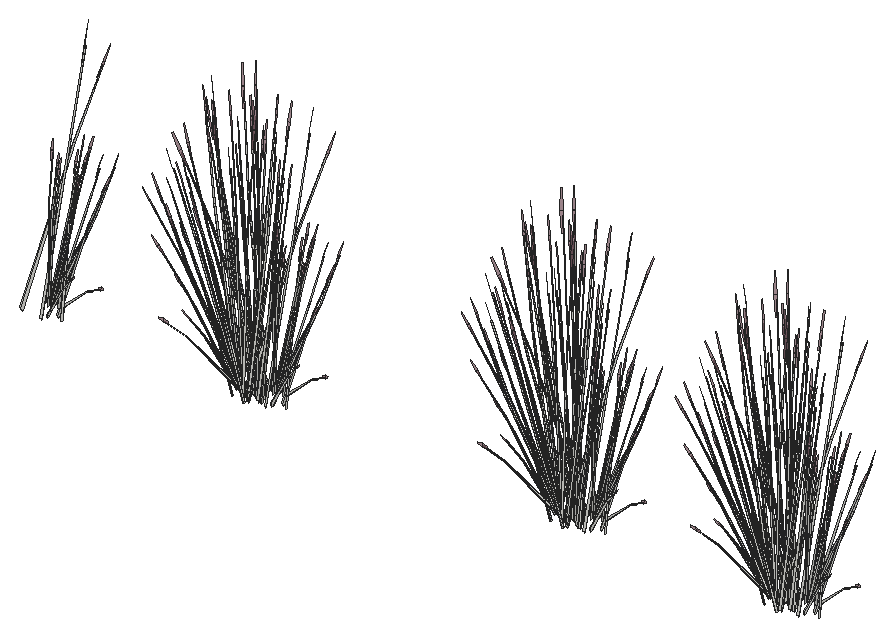
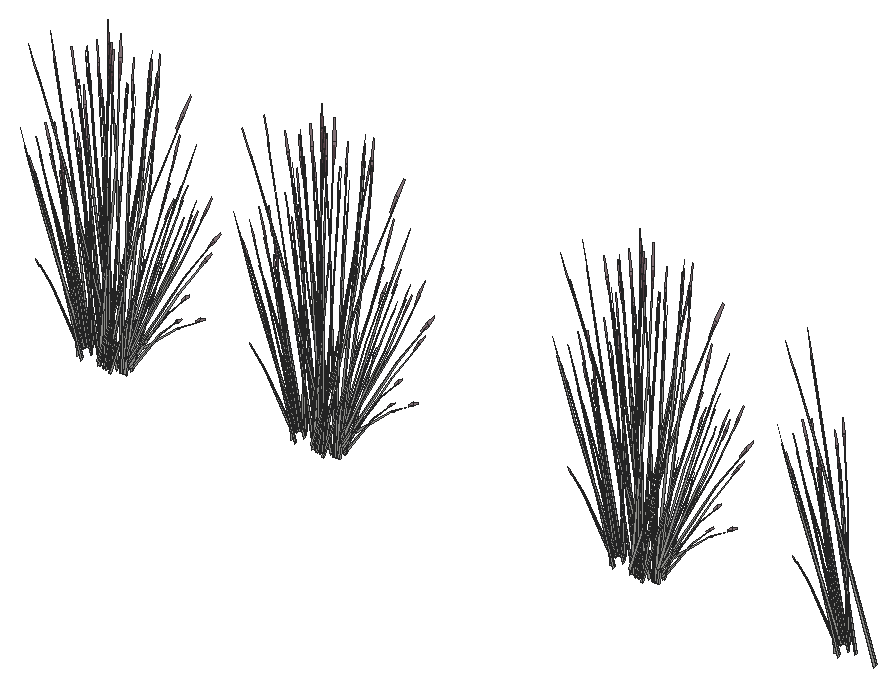
# SketchUp Ruby script. Lengths in inches.
U = 1.inch
M = Sketchup.active_model
def pt(a) = Geom::Point3d.new(a.map { |v| v * U })
def face(e, loops, mat)
  f = e.add_face(loops[0].map { |a| pt(a) })
  loops[1..].each { |l| e.add_face(l.map { |a| pt(a) }).erase! }
  f.material = f.back_material = mat if mat
  f
end
# faces: each face lists its corners as indices into pts; further lists are holes
def faces(e, pts, list, mat = nil) = list.each { |f| face(e, (f[0].is_a?(Array) ? f : [f]).map { |l| l.map { |i| pts[i] } }, mat) }
# xy, xz, yz: faces in a plane at the given z, y or x. An outline is a flat list of corners, or four numbers for a rectangle; further outlines are holes
def ring(l) = l.size == 4 ? [[l[0], l[1]], [l[2], l[1]], [l[2], l[3]], [l[0], l[3]]] : l.each_slice(2).to_a
def flat(e, list, mat, &to3) = list.each { |f| face(e, (f[0].is_a?(Array) ? f : [f]).map { |l| ring(l).map { |u, v| to3.(u, v) } }, mat) }
def xy(e, z, list, mat = nil) = flat(e, list, mat) { |x, y| [x, y, z] }
def xz(e, y, list, mat = nil) = flat(e, list, mat) { |x, z| [x, y, z] }
def yz(e, x, list, mat = nil) = flat(e, list, mat) { |y, z| [x, y, z] }
def lines(e, pts, list) = list.each { |a, b| e.add_line(pt(pts[a]), pt(pts[b])) }
# prism: a flat outline (further loops are holes) pulled along v
def prism(e, loops, v, mat = nil)
  f = face(e, loops, mat); d = Geom::Vector3d.new(v.map { |x| x * U })
  f.pushpull(f.normal.samedirection?(d) ? d.length : -d.length)
end
def box(e, o, s, mat = nil) = prism(e, [[o, [o[0] + s[0], o[1], o[2]], [o[0] + s[0], o[1] + s[1], o[2]], [o[0], o[1] + s[1], o[2]]]], [0, 0, s[2]], mat)
def at(x, y, z, deg = 0) = Geom::Transformation.translation(pt([x, y, z])) * Geom::Transformation.rotation(ORIGIN, Z_AXIS, deg.degrees)
def axes(o, x, y, z) = Geom::Transformation.new([*x, 0, *y, 0, *z, 0, *pt(o).to_a, 1])
def part(name) = M.definitions.add(name)
# library, detail: a bought-in or finely detailed component or shape, given as its bounding box
def library(name, o, s) = part(name).tap { |d| box(d.entities, o, s) }
def detail(e, o, s) = box(e.add_group.entities, o, s)
def put(e, d, t, mat = nil) = e.add_instance(d, t).tap { |i| i.material = mat if mat }
def group(e, t, mat = nil) = e.add_group.tap { |g| g.transformation = t; g.material = mat if mat }.entities
root = M.entities
M.materials.add("LightPink_Translucent").color = [144, 107, 117]
M.materials["LightPink_Translucent"].alpha = 0.75
c1 = part("blade")
p = [[2.15,0.21,22],[0,0.17,0],[0.09,0.45,0],[2.18,0.31,22],[2.29,0.31,22],[0.38,0.45,0],
  [2.48,0.24,33],[2.49,0.24,33],[2.48,0.22,33]]
faces(c1.entities,p,[[0,1,2,3],[4,5,2,3],[6,3,4,7],[8,0,3,6]])
c2 = part("seeds")
p = [[0.3,-0.1,1.38],[-0.01,-0.03,1.59],[-0.01,-0.03,0.03],[0.14,-0.07,-0.07],[0.29,-0.03,3],[0.15,0.01,3.11]]
faces(c2.entities,p,[[0,1,2,3],[1,0,4,5]],"LightPink_Translucent")
c3 = part("blade with seeds")
put(c3.entities,c1,at(0,0,0))
put(c3.entities,c2,axes([2.4,0.25,30.99],[1.5799,-0.05474,1.17369],[-0.12525,1.92788,0.29478],[-0.07173,-0.02425,1.56792]))
put(root,c3,axes([842.6875,480.84,4.49],[0.24005,-0.25798,-0.35523],[0.42065,0.18334,0.04287],[0.14333,-0.09347,0.5025]))
put(root,c3,axes([783.8125,480.08,3.1875],[-0.28732,-0.32763,0],[0.4807,-0.18271,-0.25804],[0.10948,-0.04161,0.81856]))
put(root,c3,axes([817.51,480.08,3.1875],[-0.28732,-0.32763,0],[0.4807,-0.18271,-0.25804],[0.10948,-0.04161,0.81856]))
put(root,c3,axes([840.09,480.08,3.1875],[-0.28732,-0.32763,0],[0.4807,-0.18271,-0.25804],[0.10948,-0.04161,0.81856]))
put(root,c3,axes([762.63,480.72,4.34],[-0.11806,-0.29854,-0.25549],[0.44709,-0.05222,-0.1979],[0.12812,-0.08019,0.48886]))
put(root,c3,axes([786.4,480.72,4.34],[-0.11806,-0.29854,-0.25549],[0.44709,-0.05222,-0.1979],[0.12812,-0.08019,0.48886]))
put(root,c3,axes([820.09,480.72,4.34],[-0.11806,-0.29854,-0.25549],[0.44709,-0.05222,-0.1979],[0.12812,-0.08019,0.48886]))
put(root,c3,axes([842.68,480.72,4.34],[-0.11806,-0.29854,-0.25549],[0.44709,-0.05222,-0.1979],[0.12812,-0.08019,0.48886]))
put(root,c3,axes([784.44,479.69,3.0625],[-0.31757,0.18757,-0.01946],[-0.29098,-0.20543,-0.08825],[-0.02049,-0.05821,0.29107]))
put(root,c3,axes([818.14,479.69,3.0625],[-0.31757,0.18757,-0.01946],[-0.29098,-0.20543,-0.08825],[-0.02049,-0.05821,0.29107]))
put(root,c3,axes([840.72,479.69,3.0625],[-0.31757,0.18757,-0.01946],[-0.29098,-0.20543,-0.08825],[-0.02049,-0.05821,0.29107]))
put(root,c3,axes([782.87,479.78,4.36],[-0.09888,-0.00231,0.87472],[-0.3148,0.23079,-0.13834],[-0.16797,-0.04716,0.07015]))
put(root,c3,axes([816.57,479.78,4.36],[-0.09888,-0.00231,0.87472],[-0.3148,0.23079,-0.13834],[-0.16797,-0.04716,0.07015]))
put(root,c3,axes([839.15,479.78,4.36],[-0.09888,-0.00231,0.87472],[-0.3148,0.23079,-0.13834],[-0.16797,-0.04716,0.07015]))
put(root,c3,axes([762.84,480.93,4.52],[-0.4251,-0.18028,-0.0608],[0.24491,-0.26108,-0.33747],[0.1201,-0.09075,0.51278]))
put(root,c3,axes([786.61,480.93,4.52],[-0.4251,-0.18028,-0.0608],[0.24491,-0.26108,-0.33747],[0.1201,-0.09075,0.51278]))
put(root,c3,axes([820.3,480.93,4.52],[-0.4251,-0.18028,-0.0608],[0.24491,-0.26108,-0.33747],[0.1201,-0.09075,0.51278]))
put(root,c3,axes([842.89,480.93,4.52],[-0.4251,-0.18028,-0.0608],[0.24491,-0.26108,-0.33747],[0.1201,-0.09075,0.51278]))
put(root,c3,axes([784.85,481.91,3.66],[0.39713,0.13184,0.7563],[-0.38905,0.28403,0.29908],[-0.17427,-0.16834,0.63403]))
put(root,c3,axes([818.55,481.91,3.66],[0.39713,0.13184,0.7563],[-0.38905,0.28403,0.29908],[-0.17427,-0.16834,0.63403]))
put(root,c3,axes([841.13,481.91,3.66],[0.39713,0.13184,0.7563],[-0.38905,0.28403,0.29908],[-0.17427,-0.16834,0.63403]))
put(root,c3,axes([784.02,480.13,4.53],[0.07098,0.26335,0.17707],[-0.40574,0.06954,-0.2286],[-0.10898,-0.07547,0.4374]))
put(root,c3,axes([817.71,480.13,4.53],[0.07098,0.26335,0.17707],[-0.40574,0.06954,-0.2286],[-0.10898,-0.07547,0.4374]))
put(root,c3,axes([840.3,480.13,4.53],[0.07098,0.26335,0.17707],[-0.40574,0.06954,-0.2286],[-0.10898,-0.07547,0.4374]))
put(root,c3,axes([782.77,481,3.01],[0,-0.32696,-0.24825],[0.51416,0,0],[0,-0.07447,0.78752]))
put(root,c3,axes([816.47,481,3.01],[0,-0.32696,-0.24825],[0.51416,0,0],[0,-0.07447,0.78752]))
put(root,c3,axes([839.06,481,3.01],[0,-0.32696,-0.24825],[0.51416,0,0],[0,-0.07447,0.78752]))
put(root,c3,axes([784.2,480.03,3.01],[0.4301,-0.16348,-0.24825],[0.25708,0.29314,0],[0.09796,-0.03723,0.78752]))
put(root,c3,axes([817.9,480.03,3.01],[0.4301,-0.16348,-0.24825],[0.25708,0.29314,0],[0.09796,-0.03723,0.78752]))
put(root,c3,axes([840.48,480.03,3.01],[0.4301,-0.16348,-0.24825],[0.25708,0.29314,0],[0.09796,-0.03723,0.78752]))
put(root,c3,axes([762.99,480.6,3.3],[-0.16417,-0.00968,0.71501],[-0.16819,-0.25979,-0.15377],[0.20169,-0.07349,0.3057]))
put(root,c3,axes([786.75,480.6,3.3],[-0.16417,-0.00968,0.71501],[-0.16819,-0.25979,-0.15377],[0.20169,-0.07349,0.3057]))
put(root,c3,axes([820.45,480.6,3.3],[-0.16417,-0.00968,0.71501],[-0.16819,-0.25979,-0.15377],[0.20169,-0.07349,0.3057]))
put(root,c3,axes([843.04,480.6,3.3],[-0.16417,-0.00968,0.71501],[-0.16819,-0.25979,-0.15377],[0.20169,-0.07349,0.3057]))
put(root,c3,axes([782.8,480.3,4.55],[0.37952,-0.24129,0.26881],[0.32731,0.25625,0.22165],[-0.17806,-0.04451,0.55625]))
put(root,c3,axes([816.49,480.3,4.55],[0.37952,-0.24129,0.26881],[0.32731,0.25625,0.22165],[-0.17806,-0.04451,0.55625]))
put(root,c3,axes([839.08,480.3,4.55],[0.37952,-0.24129,0.26881],[0.32731,0.25625,0.22165],[-0.17806,-0.04451,0.55625]))
put(root,c3,axes([763.89,480.85,4.35],[-0.06002,-0.00248,0.88692],[-0.24926,-0.26607,-0.08381],[0.1001,-0.08748,0.15695]))
put(root,c3,axes([787.65,480.85,4.35],[-0.06002,-0.00248,0.88692],[-0.24926,-0.26607,-0.08381],[0.1001,-0.08748,0.15695]))
put(root,c3,axes([821.35,480.85,4.35],[-0.06002,-0.00248,0.88692],[-0.24926,-0.26607,-0.08381],[0.1001,-0.08748,0.15695]))
put(root,c3,axes([843.93,480.85,4.35],[-0.06002,-0.00248,0.88692],[-0.24926,-0.26607,-0.08381],[0.1001,-0.08748,0.15695]))
put(root,c3,axes([784.71,480.7,3.03],[0.30954,-0.24575,-0.31177],[0.38452,0.22284,-0.08182],[0.12404,-0.0613,0.68817]))
put(root,c3,axes([818.41,480.7,3.03],[0.30954,-0.24575,-0.31177],[0.38452,0.22284,-0.08182],[0.12404,-0.0613,0.68817]))
put(root,c3,axes([840.99,480.7,3.03],[0.30954,-0.24575,-0.31177],[0.38452,0.22284,-0.08182],[0.12404,-0.0613,0.68817]))
put(root,c3,axes([763.18,480.12,3.38],[-0.15307,0.16644,0.5743],[-0.13157,-0.22361,0.42196],[0.12643,-0.05603,0.12649]))
put(root,c3,axes([786.94,480.12,3.38],[-0.15307,0.16644,0.5743],[-0.13157,-0.22361,0.42196],[0.12643,-0.05603,0.12649]))
put(root,c3,axes([820.64,480.12,3.38],[-0.15307,0.16644,0.5743],[-0.13157,-0.22361,0.42196],[0.12643,-0.05603,0.12649]))
put(root,c3,axes([843.23,480.12,3.38],[-0.15307,0.16644,0.5743],[-0.13157,-0.22361,0.42196],[0.12643,-0.05603,0.12649]))
put(root,c3,axes([762.96,480.75,4.26],[0.40003,-0.04673,-0.17707],[0.10563,0.26712,0.2286],[0.11464,-0.07175,0.4374]))
put(root,c3,axes([786.73,480.75,4.26],[0.40003,-0.04673,-0.17707],[0.10563,0.26712,0.2286],[0.11464,-0.07175,0.4374]))
put(root,c3,axes([820.42,480.75,4.26],[0.40003,-0.04673,-0.17707],[0.10563,0.26712,0.2286],[0.11464,-0.07175,0.4374]))
put(root,c3,axes([843.01,480.75,4.26],[0.40003,-0.04673,-0.17707],[0.10563,0.26712,0.2286],[0.11464,-0.07175,0.4374]))
put(root,c3,axes([782.97,480.3,4.37],[0.02314,-0.24862,0.03215],[0.34943,0.00682,0.2531],[-0.13385,-0.02602,0.38595]))
put(root,c3,axes([816.67,480.3,4.37],[0.02314,-0.24862,0.03215],[0.34943,0.00682,0.2531],[-0.13385,-0.02602,0.38595]))
put(root,c3,axes([839.25,480.3,4.37],[0.02314,-0.24862,0.03215],[0.34943,0.00682,0.2531],[-0.13385,-0.02602,0.38595]))
put(root,c3,axes([784.17,481.14,3.11],[0.22297,-0.29461,-0.2237],[0.4633,0.14179,0.10766],[0,-0.06791,0.71822]))
put(root,c3,axes([817.87,481.14,3.11],[0.22297,-0.29461,-0.2237],[0.4633,0.14179,0.10766],[0,-0.06791,0.71822]))
put(root,c3,axes([840.45,481.14,3.11],[0.22297,-0.29461,-0.2237],[0.4633,0.14179,0.10766],[0,-0.06791,0.71822]))
put(root,c3,axes([782.84,480.38,4.26],[-0.26148,-0.20471,-0.17707],[0.29857,-0.19378,0.2286],[-0.1517,-0.02948,0.4374]))
put(root,c3,axes([816.53,480.38,4.26],[-0.26148,-0.20471,-0.17707],[0.29857,-0.19378,0.2286],[-0.1517,-0.02948,0.4374]))
put(root,c3,axes([839.12,480.38,4.26],[-0.26148,-0.20471,-0.17707],[0.29857,-0.19378,0.2286],[-0.1517,-0.02948,0.4374]))
put(root,c3,axes([784.375,480.99,3.33],[-0.05355,-0.37308,-0.14548],[0.55775,-0.02256,-0.25001],[0.09822,-0.04969,0.79854]))
put(root,c3,axes([818.07,480.99,3.33],[-0.05355,-0.37308,-0.14548],[0.55775,-0.02256,-0.25001],[0.09822,-0.04969,0.79854]))
put(root,c3,axes([840.66,480.99,3.33],[-0.05355,-0.37308,-0.14548],[0.55775,-0.02256,-0.25001],[0.09822,-0.04969,0.79854]))
put(root,c3,axes([782.99,481.01,3.01],[0.32079,-0.20399,-0.15489],[0.32079,0.20399,0.15489],[0,-0.06571,0.69487]))
put(root,c3,axes([816.6875,481.01,3.01],[0.32079,-0.20399,-0.15489],[0.32079,0.20399,0.15489],[0,-0.06571,0.69487]))
put(root,c3,axes([839.28,481.01,3.01],[0.32079,-0.20399,-0.15489],[0.32079,0.20399,0.15489],[0,-0.06571,0.69487]))
put(root,c3,axes([782.86,480.03,3.0625],[-0.13257,0.26698,-0.01946],[-0.40802,-0.08212,-0.08825],[-0.06195,-0.04367,0.29107]))
put(root,c3,axes([816.56,480.03,3.0625],[-0.13257,0.26698,-0.01946],[-0.40802,-0.08212,-0.08825],[-0.06195,-0.04367,0.29107]))
put(root,c3,axes([839.15,480.03,3.0625],[-0.13257,0.26698,-0.01946],[-0.40802,-0.08212,-0.08825],[-0.06195,-0.04367,0.29107]))
put(root,c3,axes([762.64,480.9,4.53],[-0.40003,0.04673,0.17707],[-0.10563,-0.26712,-0.2286],[0.11464,-0.07175,0.4374]))
put(root,c3,axes([786.4,480.9,4.53],[-0.40003,0.04673,0.17707],[-0.10563,-0.26712,-0.2286],[0.11464,-0.07175,0.4374]))
put(root,c3,axes([820.09,480.9,4.53],[-0.40003,0.04673,0.17707],[-0.10563,-0.26712,-0.2286],[0.11464,-0.07175,0.4374]))
put(root,c3,axes([842.68,480.9,4.53],[-0.40003,0.04673,0.17707],[-0.10563,-0.26712,-0.2286],[0.11464,-0.07175,0.4374]))
put(root,c3,axes([784.12,481.38,3.33],[-0.51755,-0.15601,-0.14548],[0.2492,-0.32927,-0.25001],[-0.01626,-0.08084,0.79854]))
put(root,c3,axes([817.8125,481.38,3.33],[-0.51755,-0.15601,-0.14548],[0.2492,-0.32927,-0.25001],[-0.01626,-0.08084,0.79854]))
put(root,c3,axes([840.4,481.38,3.33],[-0.51755,-0.15601,-0.14548],[0.2492,-0.32927,-0.25001],[-0.01626,-0.08084,0.79854]))
put(root,c3,axes([782.65,481.25,3.1875],[-0.57465,0,0],[0,-0.36542,-0.25804],[0,-0.08323,0.81856]))
put(root,c3,axes([816.34,481.25,3.1875],[-0.57465,0,0],[0,-0.36542,-0.25804],[0,-0.08323,0.81856]))
put(root,c3,axes([838.93,481.25,3.1875],[-0.57465,0,0],[0,-0.36542,-0.25804],[0,-0.08323,0.81856]))
put(root,c3,axes([782.74,480.6,3.3],[0.08973,0.09103,0.71501],[-0.20675,0.24743,-0.15377],[-0.2123,-0.05914,0.3057]))
put(root,c3,axes([816.4375,480.6,3.3],[0.08973,0.09103,0.71501],[-0.20675,0.24743,-0.15377],[-0.2123,-0.05914,0.3057]))
put(root,c3,axes([839.02,480.6,3.3],[0.08973,0.09103,0.71501],[-0.20675,0.24743,-0.15377],[-0.2123,-0.05914,0.3057]))
put(root,c3,axes([784.3,480.16,3.01],[0.42874,0.0809,-0.15489],[-0.10795,0.28489,0.15489],[0.08643,-0.03285,0.69487]))
put(root,c3,axes([818,480.16,3.01],[0.42874,0.0809,-0.15489],[-0.10795,0.28489,0.15489],[0.08643,-0.03285,0.69487]))
put(root,c3,axes([840.58,480.16,3.01],[0.42874,0.0809,-0.15489],[-0.10795,0.28489,0.15489],[0.08643,-0.03285,0.69487]))
put(root,c3,axes([783.11,480.52,4.49],[-0.45939,-0.00787,-0.35523],[0.03085,-0.3315,0.04287],[-0.19462,-0.03498,0.5025]))
put(root,c3,axes([816.81,480.52,4.49],[-0.45939,-0.00787,-0.35523],[0.03085,-0.3315,0.04287],[-0.19462,-0.03498,0.5025]))
put(root,c3,axes([839.4,480.52,4.49],[-0.45939,-0.00787,-0.35523],[0.03085,-0.3315,0.04287],[-0.19462,-0.03498,0.5025]))
put(root,c3,axes([763,480.86,4.37],[0.31549,0.13751,0.03215],[-0.18368,0.19581,0.2531],[0.10115,-0.06331,0.38595]))
put(root,c3,axes([786.76,480.86,4.37],[0.31549,0.13751,0.03215],[-0.18368,0.19581,0.2531],[0.10115,-0.06331,0.38595]))
put(root,c3,axes([820.46,480.86,4.37],[0.31549,0.13751,0.03215],[-0.18368,0.19581,0.2531],[0.10115,-0.06331,0.38595]))
put(root,c3,axes([843.04,480.86,4.37],[0.31549,0.13751,0.03215],[-0.18368,0.19581,0.2531],[0.10115,-0.06331,0.38595]))
put(root,c3,axes([762.91,480.8,4.37],[0.11397,0.30091,0.24001],[-0.44709,0.05222,0.1979],[0.13177,-0.07077,0.49665]))
put(root,c3,axes([786.67,480.8,4.37],[0.11397,0.30091,0.24001],[-0.44709,0.05222,0.1979],[0.13177,-0.07077,0.49665]))
put(root,c3,axes([820.37,480.8,4.37],[0.11397,0.30091,0.24001],[-0.44709,0.05222,0.1979],[0.13177,-0.07077,0.49665]))
put(root,c3,axes([842.95,480.8,4.37],[0.11397,0.30091,0.24001],[-0.44709,0.05222,0.1979],[0.13177,-0.07077,0.49665]))
put(root,c3,axes([764.12,481.17,4.36],[0.06377,-0.0498,0.87472],[-0.08162,-0.30549,-0.13834],[0.16001,-0.05792,0.07015]))
put(root,c3,axes([787.88,481.17,4.36],[0.06377,-0.0498,0.87472],[-0.08162,-0.30549,-0.13834],[0.16001,-0.05792,0.07015]))
put(root,c3,axes([821.57,481.17,4.36],[0.06377,-0.0498,0.87472],[-0.08162,-0.30549,-0.13834],[0.16001,-0.05792,0.07015]))
put(root,c3,axes([844.16,481.17,4.36],[0.06377,-0.0498,0.87472],[-0.08162,-0.30549,-0.13834],[0.16001,-0.05792,0.07015]))
put(root,c3,axes([783.09,481.15,3.17],[-0.42746,0.27488,0.15378],[-0.42772,-0.27199,-0.18246],[-0.01493,-0.07806,0.82443]))
put(root,c3,axes([816.79,481.15,3.17],[-0.42746,0.27488,0.15378],[-0.42772,-0.27199,-0.18246],[-0.01493,-0.07806,0.82443]))
put(root,c3,axes([839.37,481.15,3.17],[-0.42746,0.27488,0.15378],[-0.42772,-0.27199,-0.18246],[-0.01493,-0.07806,0.82443]))
put(root,c3,axes([782.49,479.98,4.35],[0.03407,0.03263,0.88692],[-0.16424,0.29331,-0.08381],[-0.16634,0.00212,0.15695]))
put(root,c3,axes([816.19,479.98,4.35],[0.03407,0.03263,0.88692],[-0.16424,0.29331,-0.08381],[-0.16634,0.00212,0.15695]))
put(root,c3,axes([838.77,479.98,4.35],[0.03407,0.03263,0.88692],[-0.16424,0.29331,-0.08381],[-0.16634,0.00212,0.15695]))
put(root,c3,axes([784.45,481.28,3.22],[0.5178,0.15847,0.12032],[-0.2492,0.32927,0.25001],[0,-0.0759,0.80271]))
put(root,c3,axes([818.14,481.28,3.22],[0.5178,0.15847,0.12032],[-0.2492,0.32927,0.25001],[0,-0.0759,0.80271]))
put(root,c3,axes([840.73,481.28,3.22],[0.5178,0.15847,0.12032],[-0.2492,0.32927,0.25001],[0,-0.0759,0.80271]))
put(root,c3,axes([784.25,481.73,3.22],[0.1218,-0.38743,-0.11714],[0.57753,0.06753,0.25635],[-0.10091,-0.0535,0.7822]))
put(root,c3,axes([817.94,481.73,3.22],[0.1218,-0.38743,-0.11714],[0.57753,0.06753,0.25635],[-0.10091,-0.0535,0.7822]))
put(root,c3,axes([840.53,481.73,3.22],[0.1218,-0.38743,-0.11714],[0.57753,0.06753,0.25635],[-0.10091,-0.0535,0.7822]))
put(root,c3,axes([782.96,480.58,4.34],[-0.3337,0.21658,-0.25549],[-0.29224,-0.22879,-0.1979],[-0.16955,-0.03295,0.48886]))
put(root,c3,axes([816.66,480.58,4.34],[-0.3337,0.21658,-0.25549],[-0.29224,-0.22879,-0.1979],[-0.16955,-0.03295,0.48886]))
put(root,c3,axes([839.24,480.58,4.34],[-0.3337,0.21658,-0.25549],[-0.29224,-0.22879,-0.1979],[-0.16955,-0.03295,0.48886]))
put(root,c3,axes([783.21,480.49,4.53],[0.26148,0.20471,0.17707],[-0.29857,0.19378,-0.2286],[-0.1517,-0.02948,0.4374]))
put(root,c3,axes([816.9,480.49,4.53],[0.26148,0.20471,0.17707],[-0.29857,0.19378,-0.2286],[-0.1517,-0.02948,0.4374]))
put(root,c3,axes([839.49,480.49,4.53],[0.26148,0.20471,0.17707],[-0.29857,0.19378,-0.2286],[-0.1517,-0.02948,0.4374]))
put(root,c3,axes([782.21,480.87,3.38],[0.2934,-0.0234,0.5743],[-0.18611,0.20614,0.42196],[-0.14499,-0.03092,0.12649]))
put(root,c3,axes([815.9,480.87,3.38],[0.2934,-0.0234,0.5743],[-0.18611,0.20614,0.42196],[-0.14499,-0.03092,0.12649]))
put(root,c3,axes([838.49,480.87,3.38],[0.2934,-0.0234,0.5743],[-0.18611,0.20614,0.42196],[-0.14499,-0.03092,0.12649]))
put(root,c3,axes([784.28,481.0625,3.36],[-0.49904,0.02018,0.2237],[-0.04513,-0.33504,-0.10766],[0.08934,-0.03396,0.71822]))
put(root,c3,axes([817.98,481.0625,3.36],[-0.49904,0.02018,0.2237],[-0.04513,-0.33504,-0.10766],[0.08934,-0.03396,0.71822]))
put(root,c3,axes([840.5625,481.0625,3.36],[-0.49904,0.02018,0.2237],[-0.04513,-0.33504,-0.10766],[0.08934,-0.03396,0.71822]))
put(root,c3,axes([783.14,480.36,4.52],[-0.02461,0.33251,-0.0608],[-0.4659,-0.00909,-0.33747],[-0.17944,-0.0231,0.51278]))
put(root,c3,axes([816.83,480.36,4.52],[-0.02461,0.33251,-0.0608],[-0.4659,-0.00909,-0.33747],[-0.17944,-0.0231,0.51278]))
put(root,c3,axes([839.42,480.36,4.52],[-0.02461,0.33251,-0.0608],[-0.4659,-0.00909,-0.33747],[-0.17944,-0.0231,0.51278]))
put(root,c3,axes([782.99,481.31,3.24],[0,0.32696,0.24825],[-0.51416,0,0],[0,-0.07447,0.78752]))
put(root,c3,axes([816.6875,481.31,3.24],[0,0.32696,0.24825],[-0.51416,0,0],[0,-0.07447,0.78752]))
put(root,c3,axes([839.28,481.31,3.24],[0,0.32696,0.24825],[-0.51416,0,0],[0,-0.07447,0.78752]))
put(root,c3,axes([762.86,481.63,4.52],[-0.23123,-0.29606,-0.0608],[0.41039,-0.14549,-0.33747],[0.17294,-0.03906,0.51278]))
put(root,c3,axes([786.625,481.63,4.52],[-0.23123,-0.29606,-0.0608],[0.41039,-0.14549,-0.33747],[0.17294,-0.03906,0.51278]))
put(root,c3,axes([820.32,481.63,4.52],[-0.23123,-0.29606,-0.0608],[0.41039,-0.14549,-0.33747],[0.17294,-0.03906,0.51278]))
put(root,c3,axes([842.9,481.63,4.52],[-0.23123,-0.29606,-0.0608],[0.41039,-0.14549,-0.33747],[0.17294,-0.03906,0.51278]))
put(root,c3,axes([762.84,481.38,4.34],[0.1245,-0.29741,-0.25549],[0.42685,0.10194,-0.1979],[0.17186,-0.02727,0.48886]))
put(root,c3,axes([786.6,481.38,4.34],[0.1245,-0.29741,-0.25549],[0.42685,0.10194,-0.1979],[0.17186,-0.02727,0.48886]))
put(root,c3,axes([820.3,481.38,4.34],[0.1245,-0.29741,-0.25549],[0.42685,0.10194,-0.1979],[0.17186,-0.02727,0.48886]))
put(root,c3,axes([842.88,481.38,4.34],[0.1245,-0.29741,-0.25549],[0.42685,0.10194,-0.1979],[0.17186,-0.02727,0.48886]))
put(root,c3,axes([762.17,480.17,3.1875],[0.28732,-0.32763,0],[0.4807,0.18271,-0.25804],[0.10948,0.04161,0.81856]))
put(root,c3,axes([785.93,480.17,3.1875],[0.28732,-0.32763,0],[0.4807,0.18271,-0.25804],[0.10948,0.04161,0.81856]))
put(root,c3,axes([819.625,480.17,3.1875],[0.28732,-0.32763,0],[0.4807,0.18271,-0.25804],[0.10948,0.04161,0.81856]))
put(root,c3,axes([842.21,480.17,3.1875],[0.28732,-0.32763,0],[0.4807,0.18271,-0.25804],[0.10948,0.04161,0.81856]))
put(root,c3,axes([782.54,480.8125,3.9375],[0.19062,-0.00741,0.85688],[-0.12645,0.32094,0.06928],[-0.27165,-0.01985,0.36631]))
put(root,c3,axes([816.24,480.8125,3.9375],[0.19062,-0.00741,0.85688],[-0.12645,0.32094,0.06928],[-0.27165,-0.01985,0.36631]))
put(root,c3,axes([838.82,480.8125,3.9375],[0.19062,-0.00741,0.85688],[-0.12645,0.32094,0.06928],[-0.27165,-0.01985,0.36631]))
put(root,c3,axes([784.21,481.57,3.11],[-0.27607,-0.27443,-0.2237],[0.41817,-0.19325,0.10766],[-0.08934,-0.03396,0.71822]))
put(root,c3,axes([817.9,481.57,3.11],[-0.27607,-0.27443,-0.2237],[0.41817,-0.19325,0.10766],[-0.08934,-0.03396,0.71822]))
put(root,c3,axes([840.49,481.57,3.11],[-0.27607,-0.27443,-0.2237],[0.41817,-0.19325,0.10766],[-0.08934,-0.03396,0.71822]))
put(root,c3,axes([784.27,481.18,3.18],[0.1998,0.3656,0.22877],[-0.5709,0.12713,0.08977],[0.00698,-0.06718,0.79428]))
put(root,c3,axes([817.96,481.18,3.18],[0.1998,0.3656,0.22877],[-0.5709,0.12713,0.08977],[0.00698,-0.06718,0.79428]))
put(root,c3,axes([840.55,481.18,3.18],[0.1998,0.3656,0.22877],[-0.5709,0.12713,0.08977],[0.00698,-0.06718,0.79428]))
put(root,c3,axes([763.3,481.46,2.99],[-0.29599,0.03924,0.70792],[-0.04711,-0.31232,0.04052],[0.20731,-0.04727,0.40283]))
put(root,c3,axes([787.06,481.46,2.99],[-0.29599,0.03924,0.70792],[-0.04711,-0.31232,0.04052],[0.20731,-0.04727,0.40283]))
put(root,c3,axes([820.75,481.46,2.99],[-0.29599,0.03924,0.70792],[-0.04711,-0.31232,0.04052],[0.20731,-0.04727,0.40283]))
put(root,c3,axes([843.34,481.46,2.99],[-0.29599,0.03924,0.70792],[-0.04711,-0.31232,0.04052],[0.20731,-0.04727,0.40283]))
put(root,c3,axes([763.84,481.19,3.13],[-0.28491,-0.20907,-0.03244],[0.31204,-0.19157,-0.14708],[0.08842,-0.01349,0.48512]))
put(root,c3,axes([787.6,481.19,3.13],[-0.28491,-0.20907,-0.03244],[0.31204,-0.19157,-0.14708],[0.08842,-0.01349,0.48512]))
put(root,c3,axes([821.29,481.19,3.13],[-0.28491,-0.20907,-0.03244],[0.31204,-0.19157,-0.14708],[0.08842,-0.01349,0.48512]))
put(root,c3,axes([843.88,481.19,3.13],[-0.28491,-0.20907,-0.03244],[0.31204,-0.19157,-0.14708],[0.08842,-0.01349,0.48512]))
put(root,c3,axes([784.16,481.47,3.36],[-0.22297,0.29461,0.2237],[-0.4633,-0.14179,-0.10766],[0,-0.06791,0.71822]))
put(root,c3,axes([817.86,481.47,3.36],[-0.22297,0.29461,0.2237],[-0.4633,-0.14179,-0.10766],[0,-0.06791,0.71822]))
put(root,c3,axes([840.45,481.47,3.36],[-0.22297,0.29461,0.2237],[-0.4633,-0.14179,-0.10766],[0,-0.06791,0.71822]))
put(root,c3,axes([784.98,481.21,3.1],[0,-0.37831,0],[0.57465,0,0],[0,0,0.89728]))
put(root,c3,axes([818.68,481.21,3.1],[0,-0.37831,0],[0.57465,0,0],[0,0,0.89728]))
put(root,c3,axes([841.27,481.21,3.1],[0,-0.37831,0],[0.57465,0,0],[0,0,0.89728]))
put(root,c3,axes([785.68,480.34,3.24],[-0.4301,-0.16348,0.24825],[0.25708,-0.29314,0],[0.09796,0.03723,0.78752]))
put(root,c3,axes([819.375,480.34,3.24],[-0.4301,-0.16348,0.24825],[0.25708,-0.29314,0],[0.09796,0.03723,0.78752]))
put(root,c3,axes([841.96,480.34,3.24],[-0.4301,-0.16348,0.24825],[0.25708,-0.29314,0],[0.09796,0.03723,0.78752]))
put(root,c3,axes([762.76,481.49,4.49],[0.40382,-0.1444,-0.35523],[0.22505,0.29724,0.04287],[0.19512,-0.03377,0.5025]))
put(root,c3,axes([786.52,481.49,4.49],[0.40382,-0.1444,-0.35523],[0.22505,0.29724,0.04287],[0.19512,-0.03377,0.5025]))
put(root,c3,axes([820.22,481.49,4.49],[0.40382,-0.1444,-0.35523],[0.22505,0.29724,0.04287],[0.19512,-0.03377,0.5025]))
put(root,c3,axes([842.8,481.49,4.49],[0.40382,-0.1444,-0.35523],[0.22505,0.29724,0.04287],[0.19512,-0.03377,0.5025]))
put(root,c3,axes([783.96,481.67,3.03],[-0.47805,-0.0536,-0.31177],[0.10088,-0.33065,-0.08182],[-0.14266,-0.04007,0.68817]))
put(root,c3,axes([817.66,481.67,3.03],[-0.47805,-0.0536,-0.31177],[0.10088,-0.33065,-0.08182],[-0.14266,-0.04007,0.68817]))
put(root,c3,axes([840.24,481.67,3.03],[-0.47805,-0.0536,-0.31177],[0.10088,-0.33065,-0.08182],[-0.14266,-0.04007,0.68817]))
put(root,c3,axes([784.71,480.97,3.18],[-0.38104,0.29672,0.22877],[-0.45269,-0.26192,0.08977],[0.09186,-0.02961,0.79428]))
put(root,c3,axes([818.41,480.97,3.18],[-0.38104,0.29672,0.22877],[-0.45269,-0.26192,0.08977],[0.09186,-0.02961,0.79428]))
put(root,c3,axes([840.99,480.97,3.18],[-0.38104,0.29672,0.22877],[-0.45269,-0.26192,0.08977],[0.09186,-0.02961,0.79428]))
put(root,c3,axes([785.13,481.51,3.15],[-0.42746,-0.28142,-0.03066],[0.42772,-0.28159,0],[-0.01493,-0.00983,0.87786]))
put(root,c3,axes([818.82,481.51,3.15],[-0.42746,-0.28142,-0.03066],[0.42772,-0.28159,0],[-0.01493,-0.00983,0.87786]))
put(root,c3,axes([841.41,481.51,3.15],[-0.42746,-0.28142,-0.03066],[0.42772,-0.28159,0],[-0.01493,-0.00983,0.87786]))
put(root,c3,axes([784.05,480.49,3.24],[-0.13276,0.32494,0.08821],[-0.4858,-0.09195,0.17543],[0.08392,-0.00158,0.80203]))
put(root,c3,axes([817.75,480.49,3.24],[-0.13276,0.32494,0.08821],[-0.4858,-0.09195,0.17543],[0.08392,-0.00158,0.80203]))
put(root,c3,axes([840.33,480.49,3.24],[-0.13276,0.32494,0.08821],[-0.4858,-0.09195,0.17543],[0.08392,-0.00158,0.80203]))
put(root,c3,axes([762.7,481.54,4.53],[-0.38192,-0.09121,0.17707],[0.11139,-0.2661,-0.2286],[0.15377,-0.0244,0.4374]))
put(root,c3,axes([786.46,481.54,4.53],[-0.38192,-0.09121,0.17707],[0.11139,-0.2661,-0.2286],[0.15377,-0.0244,0.4374]))
put(root,c3,axes([820.16,481.54,4.53],[-0.38192,-0.09121,0.17707],[0.11139,-0.2661,-0.2286],[0.15377,-0.0244,0.4374]))
put(root,c3,axes([842.74,481.54,4.53],[-0.38192,-0.09121,0.17707],[0.11139,-0.2661,-0.2286],[0.15377,-0.0244,0.4374]))
put(root,c3,axes([782.46,481.06,4.37],[0.12984,-0.29812,0.24001],[0.42685,0.10194,0.1979],[-0.16786,0.01792,0.49665]))
put(root,c3,axes([816.16,481.06,4.37],[0.12984,-0.29812,0.24001],[0.42685,0.10194,0.1979],[-0.16786,0.01792,0.49665]))
put(root,c3,axes([838.75,481.06,4.37],[0.12984,-0.29812,0.24001],[0.42685,0.10194,0.1979],[-0.16786,0.01792,0.49665]))
put(root,c3,axes([760.09,480.75,2.8],[-0.45234,0.1309,0.64464],[-0.14398,-0.37559,0.25048],[0.27777,0.00625,0.73321]))
put(root,c3,axes([783.85,480.75,2.8],[-0.45234,0.1309,0.64464],[-0.14398,-0.37559,0.25048],[0.27777,0.00625,0.73321]))
put(root,c3,axes([817.54,480.75,2.8],[-0.45234,0.1309,0.64464],[-0.14398,-0.37559,0.25048],[0.27777,0.00625,0.73321]))
put(root,c3,axes([840.13,480.75,2.8],[-0.45234,0.1309,0.64464],[-0.14398,-0.37559,0.25048],[0.27777,0.00625,0.73321]))
put(root,c3,axes([785.06,480.85,3.31],[0.08866,-0.29179,0.0724],[0.43315,0.05065,-0.20674],[0.07883,0.02996,0.63372]))
put(root,c3,axes([818.76,480.85,3.31],[0.08866,-0.29179,0.0724],[0.43315,0.05065,-0.20674],[0.07883,0.02996,0.63372]))
put(root,c3,axes([841.35,480.85,3.31],[0.08866,-0.29179,0.0724],[0.43315,0.05065,-0.20674],[0.07883,0.02996,0.63372]))
